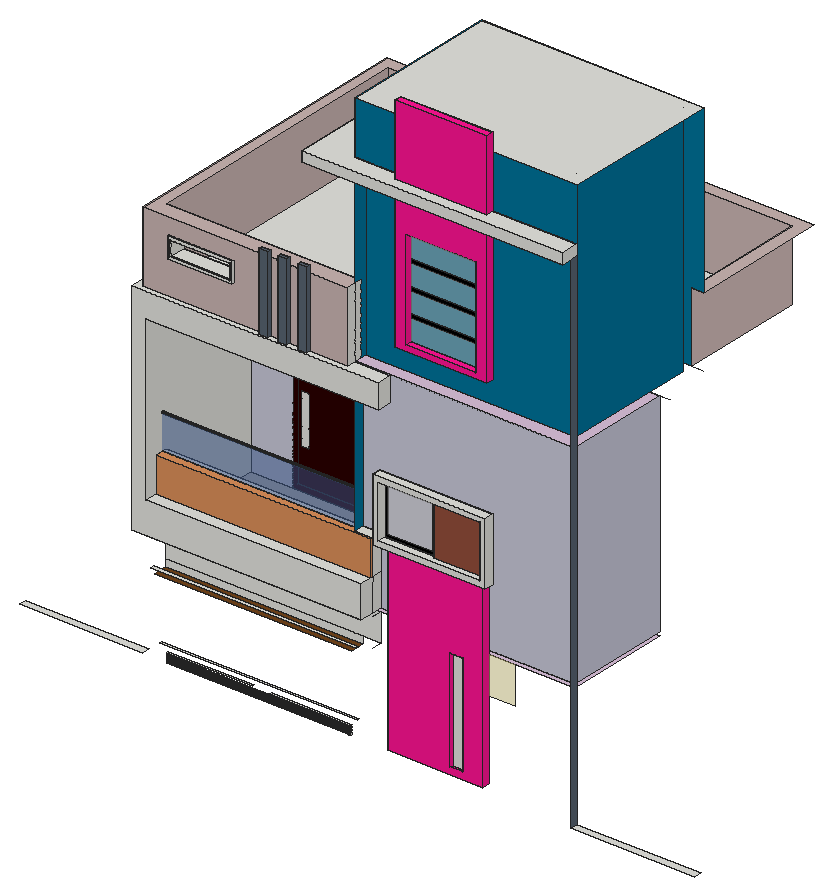
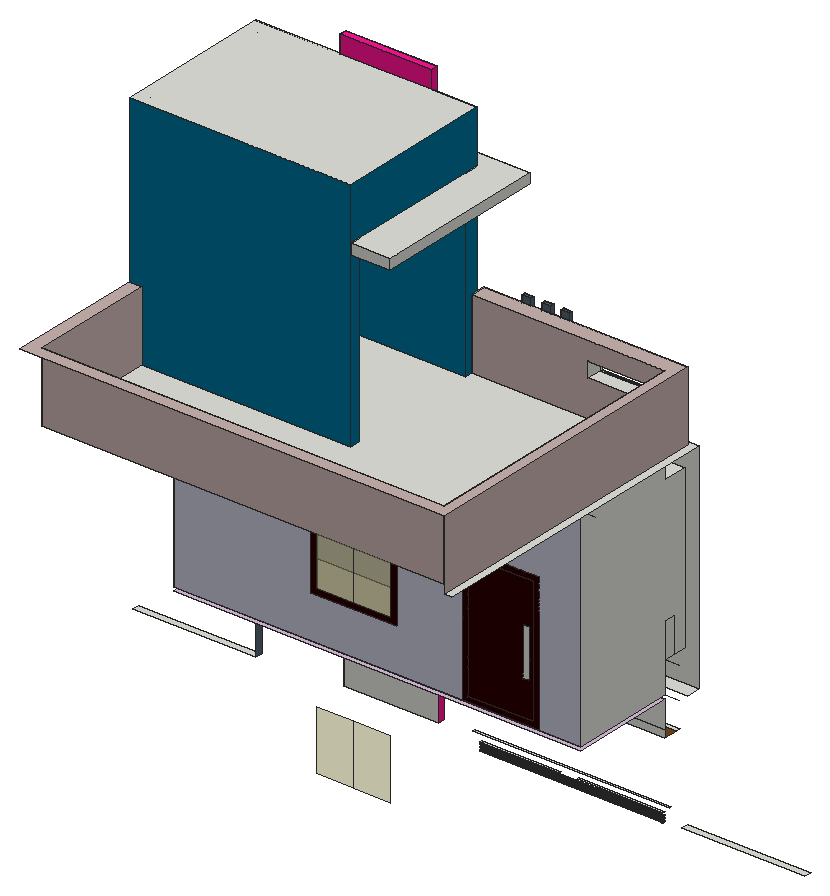
# SketchUp Ruby script. Lengths in inches.
U = 1.inch
M = Sketchup.active_model
def pt(a) = Geom::Point3d.new(a.map { |v| v * U })
def face(e, loops, mat)
  f = e.add_face(loops[0].map { |a| pt(a) })
  loops[1..].each { |l| e.add_face(l.map { |a| pt(a) }).erase! }
  f.material = f.back_material = mat if mat
  f
end
# faces: each face lists its corners as indices into pts; further lists are holes
def faces(e, pts, list, mat = nil) = list.each { |f| face(e, (f[0].is_a?(Array) ? f : [f]).map { |l| l.map { |i| pts[i] } }, mat) }
# xy, xz, yz: faces in a plane at the given z, y or x. An outline is a flat list of corners, or four numbers for a rectangle; further outlines are holes
def ring(l) = l.size == 4 ? [[l[0], l[1]], [l[2], l[1]], [l[2], l[3]], [l[0], l[3]]] : l.each_slice(2).to_a
def flat(e, list, mat, &to3) = list.each { |f| face(e, (f[0].is_a?(Array) ? f : [f]).map { |l| ring(l).map { |u, v| to3.(u, v) } }, mat) }
def xy(e, z, list, mat = nil) = flat(e, list, mat) { |x, y| [x, y, z] }
def xz(e, y, list, mat = nil) = flat(e, list, mat) { |x, z| [x, y, z] }
def yz(e, x, list, mat = nil) = flat(e, list, mat) { |y, z| [x, y, z] }
def lines(e, pts, list) = list.each { |a, b| e.add_line(pt(pts[a]), pt(pts[b])) }
# prism: a flat outline (further loops are holes) pulled along v
def prism(e, loops, v, mat = nil)
  f = face(e, loops, mat); d = Geom::Vector3d.new(v.map { |x| x * U })
  f.pushpull(f.normal.samedirection?(d) ? d.length : -d.length)
end
def box(e, o, s, mat = nil) = prism(e, [[o, [o[0] + s[0], o[1], o[2]], [o[0] + s[0], o[1] + s[1], o[2]], [o[0], o[1] + s[1], o[2]]]], [0, 0, s[2]], mat)
def at(x, y, z, deg = 0) = Geom::Transformation.translation(pt([x, y, z])) * Geom::Transformation.rotation(ORIGIN, Z_AXIS, deg.degrees)
def axes(o, x, y, z) = Geom::Transformation.new([*x, 0, *y, 0, *z, 0, *pt(o).to_a, 1])
def part(name) = M.definitions.add(name)
# library, detail: a bought-in or finely detailed component or shape, given as its bounding box
def library(name, o, s) = part(name).tap { |d| box(d.entities, o, s) }
def detail(e, o, s) = box(e.add_group.entities, o, s)
def put(e, d, t, mat = nil) = e.add_instance(d, t).tap { |i| i.material = mat if mat }
def group(e, t, mat = nil) = e.add_group.tap { |g| g.transformation = t; g.material = mat if mat }.entities
root = M.entities
M.materials.add("[0003_DeepPink]").color = [255, 20, 147]
M.materials.add("[0007_MistyRose]").color = [201, 180, 177]
M.materials.add("[0007_MistyRose]1").color = [209, 186, 184]
M.materials.add("[0022_Maroon]").color = [43, 0, 0]
M.materials.add("[0097_DeepSkyBlue]").color = [0, 114, 153]
M.materials.add("[0111_SlateGray]").color = [87, 99, 112]
M.materials.add("[0116_Lavender]").color = [199, 199, 216]
M.materials.add("[0118_Thistle]").color = [216, 191, 216]
M.materials.add("[0137_Black]").color = [0, 0, 0]
M.materials.add("[Beadboard]").color = [218, 143, 90]
M.materials.add("[Cladding Siding Tan]").color = [145, 77, 59]
M.materials.add("[Stone Vein Gray]").color = [166, 165, 165]
M.materials.add("[Translucent Glass Blue]").color = [71, 105, 168]
M.materials["[Translucent Glass Blue]"].alpha = 0.5
M.materials.add("[Translucent Glass Gray]").color = [214, 214, 214]
M.materials["[Translucent Glass Gray]"].alpha = 0.5
M.materials.add("[Translucent Glass Gray]1").color = [214, 203, 126]
M.materials["[Translucent Glass Gray]1"].alpha = 0.5
M.materials.add("[Wood Bamboo]").color = [114, 68, 27]
xy(root,342.51,[[1896,36,2316,60]])
xy(root,348,[[0,60,420,84]])
xy(root,360.11,[[1272,36,1596,60]],"[0003_DeepPink]")
xy(root,366.05,[[843.34,71.03,1116.05,78]])
xy(root,368.4,[[489.6,71.03,782.4,78]])
xy(root,382.62,[[1483.92,36,1526.36,48]],"[0003_DeepPink]")
xy(root,390,[[468,71.03,1140,78]])
xy(root,612,[[468,48,1140,96]],"[Wood Bamboo]")
xy(root,624,[[456,48,1152,60]])
xy(root,732,[[468,96,1860,455.71]],"[0118_Thistle]")
xy(root,732.43,[[1483.92,36,1526.36,48]],"[0003_DeepPink]")
xy(root,744,[[420,12,1200,60]])
xy(root,744,[[468,96,1860,455.71]],"[Stone Vein Gray]")
xy(root,852,[[468,12,1200,54],[468,54,1200,96]])
xy(root,972,[[1224,30,1224,60,1272,60,1272,36,1596,36,1596,60,1608,60,1608,30],[1272,36,1596,60],[1140,60,1200,96],[468,78,1140,96]])
xy(root,972,[[468,54,1200,54,1200,60,1140,60,1140,78,468,78]],"[Beadboard]")
xy(root,990,[[1242,30,1590,30,1590,53,1416,53,1416,60,1242,60],[1416,53,1590,60]])
xy(root,1170,[[1242,30,1242,60,1416,60,1416,53,1590,53,1590,30],[1416,53,1590,60]])
xy(root,1188,[[1224,30,1608,60]])
xy(root,1404,[[468,12,468,96,1140,96,1140,60,1260,60,1260,12]])
xy(root,1464,[[633.31,174.71,627.09,175.53,621.31,177.93,616.34,181.74,612.52,186.71,610.125,192.5,609.31,198.71,610.125,204.92,612.52,210.71,616.34,215.68,621.31,219.5,627.09,221.89,633.31,222.71,639.52,221.89,645.31,219.5,650.28,215.68,654.09,210.71,656.49,204.92,657.31,198.71,656.49,192.5,654.09,186.71,650.28,181.74,645.31,177.93,639.52,175.53],[974.56,174.71,968.34,175.53,962.56,177.93,957.59,181.74,953.77,186.71,951.375,192.5,950.56,198.71,951.375,204.92,953.77,210.71,957.59,215.68,962.56,219.5,968.34,221.89,974.56,222.71,980.77,221.89,986.56,219.5,991.53,215.68,995.34,210.71,997.74,204.92,998.56,198.71,997.74,192.5,995.34,186.71,991.53,181.74,986.56,177.93,980.77,175.53],[605.42,323.9,599.21,324.72,593.42,327.11,588.45,330.93,584.63,335.9,582.24,341.6875,581.42,347.9,582.24,354.11,584.63,359.9,588.45,364.87,593.42,368.68,599.21,371.08,605.42,371.9,611.63,371.08,617.42,368.68,622.39,364.87,626.2,359.9,628.6,354.11,629.42,347.9,628.6,341.6875,626.2,335.9,622.39,330.93,617.42,327.11,611.63,324.72],[974.56,323.9,968.34,324.72,962.56,327.11,957.59,330.93,953.77,335.9,951.375,341.6875,950.56,347.9,951.375,354.11,953.77,359.9,957.59,364.87,962.56,368.68,968.34,371.08,974.56,371.9,980.77,371.08,986.56,368.68,991.53,364.87,995.34,359.9,997.74,354.11,998.56,347.9,997.74,341.6875,995.34,335.9,991.53,330.93,986.56,327.11,980.77,324.72]])
xy(root,1464,[[[468,96,1860,455.71],[633.31,174.71,639.52,175.53,645.31,177.93,650.28,181.74,654.09,186.71,656.49,192.5,657.31,198.71,656.49,204.92,654.09,210.71,650.28,215.68,645.31,219.5,639.52,221.89,633.31,222.71,627.09,221.89,621.31,219.5,616.34,215.68,612.52,210.71,610.125,204.92,609.31,198.71,610.125,192.5,612.52,186.71,616.34,181.74,621.31,177.93,627.09,175.53],[974.56,174.71,980.77,175.53,986.56,177.93,991.53,181.74,995.34,186.71,997.74,192.5,998.56,198.71,997.74,204.92,995.34,210.71,991.53,215.68,986.56,219.5,980.77,221.89,974.56,222.71,968.34,221.89,962.56,219.5,957.59,215.68,953.77,210.71,951.375,204.92,950.56,198.71,951.375,192.5,953.77,186.71,957.59,181.74,962.56,177.93,968.34,175.53],[974.56,323.9,980.77,324.72,986.56,327.11,991.53,330.93,995.34,335.9,997.74,341.6875,998.56,347.9,997.74,354.11,995.34,359.9,991.53,364.87,986.56,368.68,980.77,371.08,974.56,371.9,968.34,371.08,962.56,368.68,957.59,364.87,953.77,359.9,951.375,354.11,950.56,347.9,951.375,341.6875,953.77,335.9,957.59,330.93,962.56,327.11,968.34,324.72],[605.42,323.9,611.63,324.72,617.42,327.11,622.39,330.93,626.2,335.9,628.6,341.6875,629.42,347.9,628.6,354.11,626.2,359.9,622.39,364.87,617.42,368.68,611.63,371.08,605.42,371.9,599.21,371.08,593.42,368.68,588.45,364.87,584.63,359.9,582.24,354.11,581.42,347.9,582.24,341.6875,584.63,335.9,588.45,330.93,593.42,327.11,599.21,324.72]]],"[0118_Thistle]")
xy(root,1488,[[420,12,1260,12,1260,60,1140,60,1140,30,1009.76,30,1009.76,18,979.89,18,979.89,30,941.26,30,941.26,18,911.39,18,911.39,30,877.95,30,877.95,18,848.08,18,848.08,30,444,30,444,1067.41,420,1067.41],[848.08,18,877.95,30],[911.39,18,941.26,30],[979.89,18,1009.76,30],[480,84,1140,84,1140,108,1854,108,1854,563.71,1140,563.71,1140,599.71,1854,599.71,1854,1025.41,480,1025.41]])
xy(root,1598,[[1296,36,1608,60]],"[0003_DeepPink]")
xy(root,1603.66,[[530.84,24,751.13,30]])
xy(root,1611.8,[[538.99,24,742.99,30],[538.99,30,742.99,84]])
xy(root,1616,[[1332,36,1572,60]],"[0003_DeepPink]")
xy(root,1665.43,[[538.99,24,742.99,30],[538.99,30,742.99,84]])
xy(root,1673.57,[[530.84,24,751.13,30]])
xy(root,1728,[[444,30,1140,30,1140,84,480,84,480,1025.41,1854,1025.41,1854,599.71,1896,599.71,1896,1067.41,444,1067.41]],"[0007_MistyRose]")
xy(root,1750,[[848.08,18,877.95,30],[911.39,18,941.26,30],[979.89,18,1009.76,30]],"[0111_SlateGray]")
xy(root,1956,[[1332,36,1572,60]],"[0003_DeepPink]")
xy(root,2076,[[[1007.34,0,1007.34,599.71,1140,599.71,1140,563.71,1158,563.71,1158,108,1140,108,1140,60,1296,60,1296,36,1608,36,1608,60,1644,60,1644,36,1692,36,1692,38,1704,38,1704,36,1758,36,1758,38,1770,38,1770,36,1824,36,1824,38,1836,38,1836,36,1896,36,1896,0],[1748.76,7.1875,1750.02,7.22,1751.26,7.38,1752.48,7.68,1753.67,8.1,1754.8,8.64,1755.875,9.29,1756.87,10.06,1757.78,10.92,1758.6,11.875,1759.31,12.91,1759.91,14.01,1760.39,15.17,1760.75,16.38,1760.98,17.61,1761.07,18.87,1761.04,20.12,1760.88,21.37,1760.58,22.59,1760.17,23.77,1759.625,24.91,1758.97,25.98,1758.2,26.97,1757.34,27.89,1756.39,28.7,1755.35,29.41,1754.25,30.01,1753.09,30.49,1751.88,30.85,1750.65,31.08,1749.39,31.18,1748.14,31.15,1746.89,30.98,1745.67,30.6875,1744.49,30.27,1743.35,29.73,1742.28,29.07,1741.29,28.31,1740.375,27.44,1739.56,26.49,1738.85,25.45,1738.25,24.35,1737.77,23.19,1737.41,21.99,1737.18,20.75,1737.08,19.5,1737.12,18.24,1737.28,17,1737.57,15.78,1737.99,14.59,1738.53,13.46,1739.1875,12.39,1739.95,11.39,1740.82,10.48,1741.77,9.66,1742.81,8.95,1743.91,8.35,1745.07,7.87,1746.27,7.51,1747.51,7.29],[1208.26,15.36,1209.52,15.39,1210.76,15.56,1211.98,15.85,1213.17,16.27,1214.3,16.81,1215.37,17.46,1216.37,18.23,1217.28,19.09,1218.1,20.05,1218.81,21.08,1219.41,22.1875,1219.89,23.35,1220.25,24.55,1220.47,25.79,1220.57,27.04,1220.54,28.29,1220.38,29.54,1220.08,30.76,1219.67,31.95,1219.125,33.08,1218.47,34.15,1217.7,35.15,1216.84,36.06,1215.88,36.875,1214.85,37.59,1213.75,38.19,1212.59,38.67,1211.38,39.02,1210.15,39.25,1208.89,39.35,1207.64,39.32,1206.39,39.15,1205.17,38.86,1203.99,38.44,1202.85,37.9,1201.78,37.25,1200.79,36.48,1199.875,35.62,1199.06,34.66,1198.35,33.63,1197.75,32.52,1197.27,31.36,1196.91,30.16,1196.68,28.92,1196.58,27.67,1196.61,26.42,1196.78,25.17,1197.07,23.95,1197.49,22.77,1198.03,21.63,1198.6875,20.56,1199.45,19.5625,1200.32,18.65,1201.27,17.84,1202.31,17.125,1203.41,16.53,1204.57,16.04,1205.77,15.6875,1207.01,15.46],[1069.37,493.2,1072.46,493.74,1075.3,495.0625,1077.7,497.07,1079.5,499.64,1080.57,502.58,1080.85,505.7,1080.31,508.79,1078.99,511.63,1076.98,514.03,1074.41,515.83,1071.47,516.9,1068.35,517.18,1065.26,516.64,1062.42,515.32,1060.02,513.31,1058.22,510.74,1057.15,507.8,1056.87,504.68,1057.41,501.6,1058.73,498.75,1060.74,496.35,1063.31,494.55,1066.25,493.48],[1069.37,106.08,1072.46,106.62,1075.3,107.9375,1077.7,109.95,1079.5,112.51,1080.57,115.46,1080.85,118.58,1080.31,121.66,1078.99,124.5,1076.98,126.9,1074.41,128.7,1071.47,129.78,1068.35,130.06,1065.26,129.51,1062.42,128.19,1060.02,126.18,1058.22,123.62,1057.15,120.68,1056.87,117.56,1057.41,114.47,1058.73,111.63,1060.74,109.23,1063.31,107.43,1066.25,106.35],[1069.37,305.45,1072.46,305.99,1075.3,307.3125,1077.7,309.32,1079.5,311.89,1080.57,314.83,1080.85,317.95,1080.31,321.04,1078.99,323.88,1076.98,326.28,1074.41,328.08,1071.47,329.15,1068.35,329.43,1065.26,328.89,1062.42,327.57,1060.02,325.56,1058.22,322.99,1057.15,320.05,1056.87,316.93,1057.41,313.85,1058.73,311,1060.74,308.6,1063.31,306.8,1066.25,305.73]],[1748.76,7.1875,1747.51,7.29,1746.27,7.51,1745.07,7.87,1743.91,8.35,1742.81,8.95,1741.77,9.66,1740.82,10.48,1739.95,11.39,1739.1875,12.39,1738.53,13.46,1737.99,14.59,1737.57,15.78,1737.28,17,1737.12,18.24,1737.08,19.5,1737.18,20.75,1737.41,21.99,1737.77,23.19,1738.25,24.35,1738.85,25.45,1739.56,26.49,1740.375,27.44,1741.29,28.31,1742.28,29.07,1743.35,29.73,1744.49,30.27,1745.67,30.6875,1746.89,30.98,1748.14,31.15,1749.39,31.18,1750.65,31.08,1751.88,30.85,1753.09,30.49,1754.25,30.01,1755.35,29.41,1756.39,28.7,1757.34,27.89,1758.2,26.97,1758.97,25.98,1759.625,24.91,1760.17,23.77,1760.58,22.59,1760.88,21.37,1761.04,20.12,1761.07,18.87,1760.98,17.61,1760.75,16.38,1760.39,15.17,1759.91,14.01,1759.31,12.91,1758.6,11.875,1757.78,10.92,1756.87,10.06,1755.875,9.29,1754.8,8.64,1753.67,8.1,1752.48,7.68,1751.26,7.38,1750.02,7.22],[1208.26,15.36,1207.01,15.46,1205.77,15.6875,1204.57,16.04,1203.41,16.53,1202.31,17.125,1201.27,17.84,1200.32,18.65,1199.45,19.5625,1198.6875,20.56,1198.03,21.63,1197.49,22.77,1197.07,23.95,1196.78,25.17,1196.61,26.42,1196.58,27.67,1196.68,28.92,1196.91,30.16,1197.27,31.36,1197.75,32.52,1198.35,33.63,1199.06,34.66,1199.875,35.62,1200.79,36.48,1201.78,37.25,1202.85,37.9,1203.99,38.44,1205.17,38.86,1206.39,39.15,1207.64,39.32,1208.89,39.35,1210.15,39.25,1211.38,39.02,1212.59,38.67,1213.75,38.19,1214.85,37.59,1215.88,36.875,1216.84,36.06,1217.7,35.15,1218.47,34.15,1219.125,33.08,1219.67,31.95,1220.08,30.76,1220.38,29.54,1220.54,28.29,1220.57,27.04,1220.47,25.79,1220.25,24.55,1219.89,23.35,1219.41,22.1875,1218.81,21.08,1218.1,20.05,1217.28,19.09,1216.37,18.23,1215.37,17.46,1214.3,16.81,1213.17,16.27,1211.98,15.85,1210.76,15.56,1209.52,15.39],[1296,36,1608,60],[1644,36,1644,60,1896,60,1896,36,1836,36,1836,38,1824,38,1824,36,1770,36,1770,38,1758,38,1758,36,1704,36,1704,38,1692,38,1692,36],
  [1069.37,106.08,1066.25,106.35,1063.31,107.43,1060.74,109.23,1058.73,111.63,1057.41,114.47,1056.87,117.56,1057.15,120.68,1058.22,123.62,1060.02,126.18,1062.42,128.19,1065.26,129.51,1068.35,130.06,1071.47,129.78,1074.41,128.7,1076.98,126.9,1078.99,124.5,1080.31,121.66,1080.85,118.58,1080.57,115.46,1079.5,112.51,1077.7,109.95,1075.3,107.9375,1072.46,106.62],[1069.37,305.45,1066.25,305.73,1063.31,306.8,1060.74,308.6,1058.73,311,1057.41,313.85,1056.87,316.93,1057.15,320.05,1058.22,322.99,1060.02,325.56,1062.42,327.57,1065.26,328.89,1068.35,329.43,1071.47,329.15,1074.41,328.08,1076.98,326.28,1078.99,323.88,1080.31,321.04,1080.85,317.95,1080.57,314.83,1079.5,311.89,1077.7,309.32,1075.3,307.3125,1072.46,305.99],[1069.37,493.2,1066.25,493.48,1063.31,494.55,1060.74,496.35,1058.73,498.75,1057.41,501.6,1056.87,504.68,1057.15,507.8,1058.22,510.74,1060.02,513.31,1062.42,515.32,1065.26,516.64,1068.35,517.18,1071.47,516.9,1074.41,515.83,1076.98,514.03,1078.99,511.63,1080.31,508.79,1080.85,505.7,1080.57,502.58,1079.5,499.64,1077.7,497.07,1075.3,495.0625,1072.46,493.74]])
xy(root,2112,[[1007.34,0,1896,0,1896,60,1608,60,1608,36,1296,36,1296,60,1140,60,1140,599.71,1007.34,599.71],[1296,36,1608,60]])
xy(root,2268,[[1158,108,1854,563.71]])
xy(root,2292,[[1140,60,1896,599.71]])
xy(root,2352,[[1296,36,1608,60]],"[0003_DeepPink]")
xz(root,0,[[1007.34,2076,1896,2112]])
xz(root,12,[[420,744,1200,744,1200,852,468,852,468,1404,1260,1404,1260,1488,420,1488]])
xz(root,18,[[848.08,1488,877.95,1750],[911.39,1488,941.26,1750],[979.89,1488,1009.76,1750]],"[0111_SlateGray]")
xz(root,24,[[[530.84,1603.66,751.13,1673.57],[538.99,1611.8,742.99,1665.43]]])
xz(root,30,[[[1224,972,1608,1188],[1242,990,1590,1170]],[848.08,1488,877.95,1728],[911.39,1488,941.26,1728],[979.89,1488,1009.76,1728],[[530.84,1603.66,751.13,1673.57],[538.99,1611.8,742.99,1665.43]]])
xz(root,30,[[[444,1488,848.08,1728],[530.84,1603.66,751.13,1673.57]],[877.95,1488,911.39,1728],[941.26,1488,979.89,1728],[1009.76,1488,1140,1728]],"[0007_MistyRose]")
xz(root,30,[[848.08,1728,877.95,1750],[911.39,1728,941.26,1750],[979.89,1728,1009.76,1750]],"[0111_SlateGray]")
xz(root,36,[[[1272,360.11,1596,972],[1483.92,382.62,1526.36,732.43]],[[1296,1598,1608,2076],[1332,1616,1572,1956]],[1296,2112,1608,2352]],"[0003_DeepPink]")
xz(root,48,[[1483.92,382.62,1526.36,732.43]])
xz(root,53,[[1416,990,1590,1170]],"[Cladding Siding Tan]")
xz(root,54,[[468,852,1200,972]],"[Beadboard]")
xz(root,60,[[1272,360.11,1596,972],[[1224,972,1608,1188],[1242,990,1590,1170]],[1140,2076,1896,2112]])
xz(root,60,[[1296,2292,1608,2352]],"[0003_DeepPink]")
xz(root,60,[[1140,2112,1296,2292],[1608,2112,1896,2292]],"[0097_DeepSkyBlue]")
xz(root,60,[[[1242,990,1416,1170],[1253,1001,1405,1159]],[1332,1688,1572,1700],[1332,1772,1572,1784],[1332,1856,1572,1868]],"[0137_Black]")
xz(root,60,[[1253,1001,1405,1159],[1332,1616,1572,1688],[1332,1700,1572,1772],[1332,1784,1572,1856],[1332,1868,1572,1956]],"[Translucent Glass Gray]")
xz(root,78,[[468,1089,1140,1092]])
xz(root,78,[[468,972,1140,1089]],"[Translucent Glass Blue]")
xz(root,84,[[[480,1488,1140,1728],[538.99,1611.8,742.99,1665.43]]],"[0007_MistyRose]")
xz(root,96,[[468,612,1140,636],[468,636,1200,732],[468,744,1200,852],[468,852,1200,972],[468,1404,1200,1464]])
xz(root,96,[[1200,744,1200,972,1140,972,1140,1404,1200,1404,1200,1464,1860,1464,1860,744]],"[0116_Lavender]")
xz(root,108,[[1140,1488,1140,2076,1158,2076,1158,2268,1854,2268,1854,1488]],"[0097_DeepSkyBlue]")
xz(root,455.71,[[642.625,882.89,665.375,1050.27]])
xz(root,455.71,[[[611.72,744,872.28,1211.75],[629.72,762,854.28,1193.75]],[[629.72,762,854.28,1193.75],[642.625,882.89,665.375,1050.27]],[[1098.44,891.375,1390.19,1211.75],[1116.44,909.375,1372.19,1193.75]]],"[0022_Maroon]")
xz(root,455.71,[[[468,744,611.72,744,611.72,1211.75,872.28,1211.75,872.28,744,1860,744,1860,1464,468,1464],[1098.44,891.375,1390.19,1211.75]]],"[0116_Lavender]")
xz(root,455.71,[[1116.44,342.3,1244.32,549.56],[1244.32,342.3,1372.19,549.56],[1116.44,909.375,1244.32,1193.75],[1244.32,909.375,1372.19,1193.75]],"[Translucent Glass Gray]1")
xz(root,563.71,[[1140,1488,1854,1488,1854,2268,1158,2268,1158,2076,1140,2076]],"[0097_DeepSkyBlue]")
xz(root,599.71,[[1007.34,2076,1140,2112]])
xz(root,599.71,[[1140,1488,1140,2292,1896,2292,1896,1728,1854,1728,1854,1488]],"[0097_DeepSkyBlue]")
xz(root,1025.41,[[480,1488,1854,1728]],"[0007_MistyRose]")
yz(root,444,[[30,1488,1067.41,1728]],"[0007_MistyRose]")
yz(root,468,[[[96,744,455.71,744,455.71,1464,96,1464,96,1404,12,1404,12,852,54,852,54,972,96,972],[78,1089,77.22,1089.1,76.5,1089.4,75.88,1089.88,75.4,1090.5,75.1,1091.22,75,1092,75.1,1092.78,75.4,1093.5,75.88,1094.12,76.5,1094.6,77.22,1094.9,78,1095,78.78,1094.9,79.5,1094.6,80.12,1094.12,80.6,1093.5,80.9,1092.78,81,1092,80.9,1091.22,80.6,1090.5,80.12,1089.88,79.5,1089.4,78.78,1089.1]],[54,852,96,972],[78,1089,77.22,1089.1,76.5,1089.4,75.88,1089.88,75.4,1090.5,75.1,1091.22,75,1092,75.1,1092.78,75.4,1093.5,75.88,1094.12,76.5,1094.6,77.22,1094.9,78,1095,78.78,1094.9,79.5,1094.6,80.12,1094.12,80.6,1093.5,80.9,1092.78,81,1092,80.9,1091.22,80.6,1090.5,80.12,1089.88,79.5,1089.4,78.78,1089.1]])
yz(root,480,[[84,1488,1025.41,1728]],"[0007_MistyRose]")
yz(root,530.84,[[24,1603.66,30,1673.57]])
yz(root,538.99,[[24,1611.8,30,1665.43],[30,1611.8,84,1665.43]])
yz(root,742.99,[[24,1611.8,30,1665.43],[30,1611.8,84,1665.43]])
yz(root,751.13,[[24,1603.66,30,1673.57]])
yz(root,848.08,[[18,1488,30,1750]],"[0111_SlateGray]")
yz(root,877.95,[[18,1488,30,1750]],"[0111_SlateGray]")
yz(root,911.39,[[18,1488,30,1750]],"[0111_SlateGray]")
yz(root,941.26,[[18,1488,30,1750]],"[0111_SlateGray]")
yz(root,979.89,[[18,1488,30,1750]],"[0111_SlateGray]")
yz(root,1007.34,[[0,2076,599.71,2112]])
yz(root,1009.76,[[18,1488,30,1750]],"[0111_SlateGray]")
yz(root,1116.41,[[74.52,336.6875,75.03,336.75,75.52,336.95,75.93,337.27,76.25,337.6875,76.45,338.17,76.52,338.6875,76.45,339.2,76.25,339.6875,75.93,340.1,75.52,340.42,75.03,340.62,74.52,340.6875,74,340.62,73.52,340.42,73.1,340.1,72.78,339.6875,72.58,339.2,72.52,338.6875,72.58,338.17,72.78,337.6875,73.1,337.27,73.52,336.95,74,336.75]])
yz(root,1140,[[30,1488,60,1728],[60,1488,84,1728],[60,2076,108,2112],[563.71,2076,599.71,2112]])
yz(root,1140,[[[60,972,96,1404],[78,1089,78.78,1089.1,79.5,1089.4,80.12,1089.88,80.6,1090.5,80.9,1091.22,81,1092,80.9,1092.78,80.6,1093.5,80.12,1094.12,79.5,1094.6,78.78,1094.9,78,1095,77.22,1094.9,76.5,1094.6,75.88,1094.12,75.4,1093.5,75.1,1092.78,75,1092,75.1,1091.22,75.4,1090.5,75.88,1089.88,76.5,1089.4,77.22,1089.1]],[84,1488,84,1728,60,1728,60,2076,108,2076,108,1488],[563.71,1488,599.71,2076],[60,2112,599.71,2292]],"[0097_DeepSkyBlue]")
yz(root,1158,[[108,2076,563.71,2268]])
yz(root,1200,[[12,744,60,852],[60,744,96,852],[60,852,96,972]])
yz(root,1200,[[54,852,60,972]],"[Beadboard]")
yz(root,1224,[[30,972,60,1188]])
yz(root,1242,[[30,990,60,1170]])
yz(root,1260,[[12,1404,60,1488]])
yz(root,1272,[[36,360.11,60,972]],"[0003_DeepPink]")
yz(root,1296,[[36,1598,60,2076],[36,2112,60,2352]],"[0003_DeepPink]")
yz(root,1332,[[36,1616,60,1956]],"[0003_DeepPink]")
yz(root,1416,[[53,990,60,1170]])
yz(root,1483.92,[[36,382.62,48,732.43]],"[0003_DeepPink]")
yz(root,1526.36,[[36,382.62,48,732.43]],"[0003_DeepPink]")
yz(root,1572,[[36,1616,60,1956]],"[0003_DeepPink]")
yz(root,1590,[[30,990,53,1170],[53,990,60,1170]])
yz(root,1596,[[36,360.11,60,972]],"[0003_DeepPink]")
yz(root,1608,[[30,972,60,1188]])
yz(root,1608,[[36,1598,60,2076],[36,2112,60,2352]],"[0003_DeepPink]")
yz(root,1854,[[599.71,1488,1025.41,1728]],"[0007_MistyRose]1")
yz(root,1854,[[108,1488,563.71,2268]],"[0097_DeepSkyBlue]")
yz(root,1860,[[96,744,455.71,1464]],"[0116_Lavender]")
yz(root,1896,[[0,2076,60,2112]])
yz(root,1896,[[36,342.51,60,2076]],"[0111_SlateGray]")
p = [[489.6,74,336.75],[489.6,74.52,336.6875],[1116.41,74.52,336.6875],[1116.41,74,336.75],[489.6,75.03,336.75],[1116.41,75.03,336.75],
  [489.6,73.52,336.95],[1116.41,73.52,336.95],[489.6,75.52,336.95],[1116.41,75.52,336.95],[489.6,73.1,337.27],[1116.41,73.1,337.27],
  [489.6,75.93,337.27],[1116.41,75.93,337.27],[489.6,72.78,337.6875],[1116.41,72.78,337.6875],[489.6,76.25,337.6875],[1116.41,76.25,337.6875],
  [489.6,72.58,338.17],[1116.41,72.58,338.17],[489.6,76.45,338.17],[1116.41,76.45,338.17],[489.6,72.52,338.6875],[1116.41,72.52,338.6875],
  [489.6,76.52,338.6875],[1116.41,76.52,338.6875],[489.6,72.58,339.2],[1116.41,72.58,339.2],[489.6,76.45,339.2],[1116.41,76.45,339.2],
  [489.6,72.78,339.6875],[1116.41,72.78,339.6875],[489.6,76.25,339.6875],[1116.41,76.25,339.6875],[489.6,73.1,340.1],[1116.41,73.1,340.1],
  [489.6,75.93,340.1],[1116.41,75.93,340.1],[489.6,73.52,340.42],[1116.41,73.52,340.42],[489.6,75.52,340.42],[1116.41,75.52,340.42],
  [489.6,74,340.62],[1116.41,74,340.62],[489.6,75.03,340.62],[1116.41,75.03,340.62],[489.6,74.52,340.6875],[1116.41,74.52,340.6875],
  [489.6,74,346.75],[489.6,74.52,346.6875],[1116.05,74.52,346.6875],[1116.05,74,346.75],[489.6,75.03,346.75],[1116.05,75.03,346.75],
  [489.6,73.52,346.95],[1116.05,73.52,346.95],[489.6,75.52,346.95],[1116.05,75.52,346.95],[489.6,73.1,347.27],[1116.05,73.1,347.27],
  [489.6,75.93,347.27],[1116.05,75.93,347.27],[489.6,72.78,347.6875],[1116.05,72.78,347.6875],[489.6,76.25,347.6875],[1116.05,76.25,347.6875],
  [489.6,72.58,348.17],[1116.05,72.58,348.17],[489.6,76.45,348.17],[1116.05,76.45,348.17],[489.6,72.52,348.6875],[1116.05,72.52,348.6875],
  [489.6,76.52,348.6875],[1116.05,76.52,348.6875],[489.6,72.58,349.2],[1116.05,72.58,349.2],[489.6,76.45,349.2],[1116.05,76.45,349.2],
  [489.6,72.78,349.6875],[1116.05,72.78,349.6875],[489.6,76.25,349.6875],[1116.05,76.25,349.6875],[489.6,73.1,350.1],[1116.05,73.1,350.1],
  [489.6,75.93,350.1],[1116.05,75.93,350.1],[489.6,73.52,350.42],[1116.05,73.52,350.42],[489.6,75.52,350.42],[1116.05,75.52,350.42],
  [489.6,74,350.62],[1116.05,74,350.62],[489.6,75.03,350.62],[1116.05,75.03,350.62],[489.6,74.52,350.6875],[1116.05,74.52,350.6875],
  [489.6,74,356.75],[489.6,74.52,356.6875],[1116.05,74.52,356.6875],[1116.05,74,356.75],[489.6,75.03,356.75],[1116.05,75.03,356.75],
  [489.6,73.52,356.95],[1116.05,73.52,356.95],[489.6,75.52,356.95],[1116.05,75.52,356.95],[489.6,73.1,357.27],[1116.05,73.1,357.27],
  [489.6,75.93,357.27],[1116.05,75.93,357.27],[489.6,72.78,357.6875],[1116.05,72.78,357.6875],[489.6,76.25,357.6875],[1116.05,76.25,357.6875],
  [489.6,72.58,358.17],[1116.05,72.58,358.17],[489.6,76.45,358.17],[1116.05,76.45,358.17],[489.6,72.52,358.6875],[1116.05,72.52,358.6875],
  [489.6,76.52,358.6875],[1116.05,76.52,358.6875],[489.6,72.58,359.2],[1116.05,72.58,359.2],[489.6,76.45,359.2],[1116.05,76.45,359.2],
  [489.6,72.78,359.6875],[1116.05,72.78,359.6875],[489.6,76.25,359.6875],[1116.05,76.25,359.6875],[489.6,73.1,360.1],[1116.05,73.1,360.1],
  [489.6,75.93,360.1],[1116.05,75.93,360.1],[489.6,73.52,360.42],[1116.05,73.52,360.42],[489.6,75.52,360.42],[1116.05,75.52,360.42],
  [489.6,74,360.62],[1116.05,74,360.62],[489.6,75.03,360.62],[1116.05,75.03,360.62],[489.6,74.52,360.6875],[1116.05,74.52,360.6875],
  [468,77.22,1089.1],[468,78,1089],[1140,78,1089],[1140,77.22,1089.1],[468,78.78,1089.1],[1140,78.78,1089.1],
  [468,76.5,1089.4],[1140,76.5,1089.4],[468,79.5,1089.4],[1140,79.5,1089.4],[468,75.88,1089.88],[1140,75.88,1089.88],
  [468,80.12,1089.88],[1140,80.12,1089.88],[468,75.4,1090.5],[1140,75.4,1090.5],[468,80.6,1090.5],[1140,80.6,1090.5],
  [468,75.1,1091.22],[1140,75.1,1091.22],[468,80.9,1091.22],[1140,80.9,1091.22],[468,75,1092],[1140,75,1092],
  [468,81,1092],[1140,81,1092],[468,75.1,1092.78],[1140,75.1,1092.78],[468,80.9,1092.78],[1140,80.9,1092.78],
  [468,75.4,1093.5],[1140,75.4,1093.5],[468,80.6,1093.5],[1140,80.6,1093.5],[468,75.88,1094.12],[1140,75.88,1094.12],
  [468,80.12,1094.12],[1140,80.12,1094.12],[468,76.5,1094.6],[1140,76.5,1094.6],[468,79.5,1094.6],[1140,79.5,1094.6],
  [468,77.22,1094.9],[1140,77.22,1094.9],[468,78.78,1094.9],[1140,78.78,1094.9],[468,78,1095],[1140,78,1095],
  [1896,455.71,1464],[1860,455.71,1464],[1200,96,732],[1200,60,732],[1200,96,636],[1200,60,636],
  [468,455.71,636],[420,455.71,636],[468,96,744],[420,96,744],[468,455.71,1464],[420,455.71,1464],
  [468,96,852],[420,96,852],[468,96,1464],[468,60,1464],[1200,60,1464],[1200,96,1464],
  [1854,599.71,1488],[1896,599.71,1488],[1854,563.71,2268],[1854,563.71,2292],[1854,108,2268],[1854,108,2292],
  [1158,563.71,2268],[1140,563.71,2268],[1158,108,2268],[1140,108,2268]]
faces(root,p,[[0,1,2,3],[1,4,5,2],[6,0,3,7],[4,8,9,5],[10,6,7,11],[8,12,13,9],[14,10,11,15],[12,16,17,13],
  [18,14,15,19],[16,20,21,17],[22,18,19,23],[20,24,25,21],[26,22,23,27],[24,28,29,25],[30,26,27,31],[28,32,33,29],
  [34,30,31,35],[32,36,37,33],[38,34,35,39],[36,40,41,37],[42,38,39,43],[40,44,45,41],[46,42,43,47],[44,46,47,45],
  [48,49,50,51],[49,52,53,50],[54,48,51,55],[52,56,57,53],[58,54,55,59],[56,60,61,57],[62,58,59,63],[60,64,65,61],
  [66,62,63,67],[64,68,69,65],[70,66,67,71],[68,72,73,69],[74,70,71,75],[72,76,77,73],[78,74,75,79],[76,80,81,77],
  [82,78,79,83],[80,84,85,81],[86,82,83,87],[84,88,89,85],[90,86,87,91],[88,92,93,89],[94,90,91,95],[92,94,95,93],
  [96,97,98,99],[97,100,101,98],[102,96,99,103],[100,104,105,101],[106,102,103,107],[104,108,109,105],[110,106,107,111],[108,112,113,109],
  [114,110,111,115],[112,116,117,113],[118,114,115,119],[116,120,121,117],[122,118,119,123],[120,124,125,121],[126,122,123,127],[124,128,129,125],
  [130,126,127,131],[128,132,133,129],[134,130,131,135],[132,136,137,133],[138,134,135,139],[136,140,141,137],[142,138,139,143],[140,142,143,141],
  [144,145,146,147],[145,148,149,146],[150,144,147,151],[148,152,153,149],[154,150,151,155],[152,156,157,153],[158,154,155,159],[156,160,161,157],
  [162,158,159,163],[160,164,165,161],[166,162,163,167],[164,168,169,165],[170,166,167,171],[168,172,173,169],[174,170,171,175],[172,176,177,173],
  [178,174,175,179],[176,180,181,177],[182,178,179,183],[180,184,185,181],[186,182,183,187],[184,188,189,185],[190,186,187,191],[188,190,191,189]])
lines(root,p,[[192,193],[194,195],[196,197],[198,199],[200,201],[202,203],[204,205],[206,207],[208,209],[210,211],[212,213],[214,215],
  [216,217],[218,219]])
